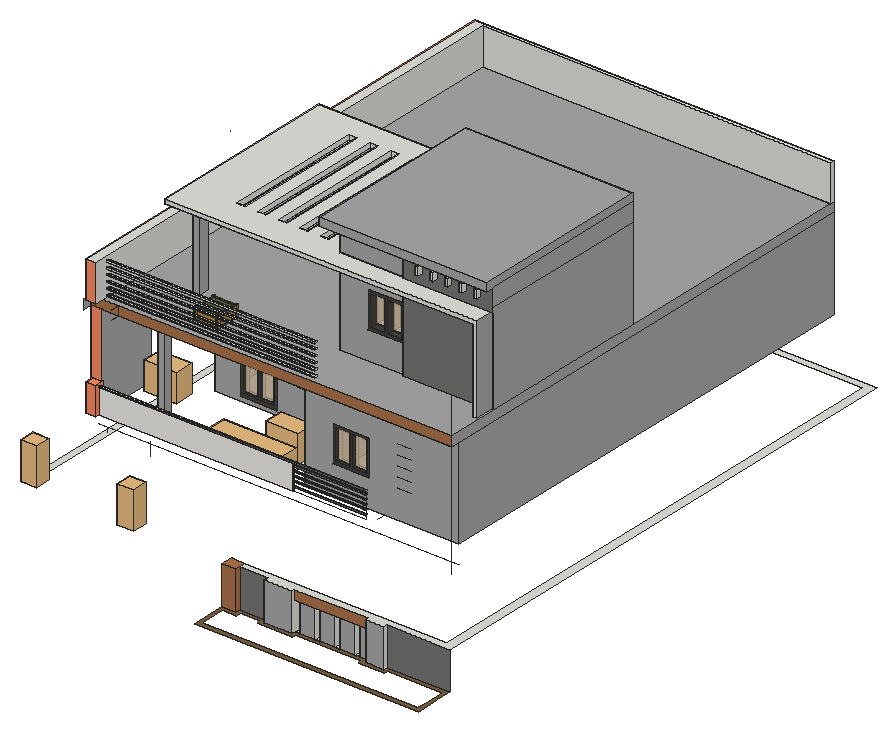
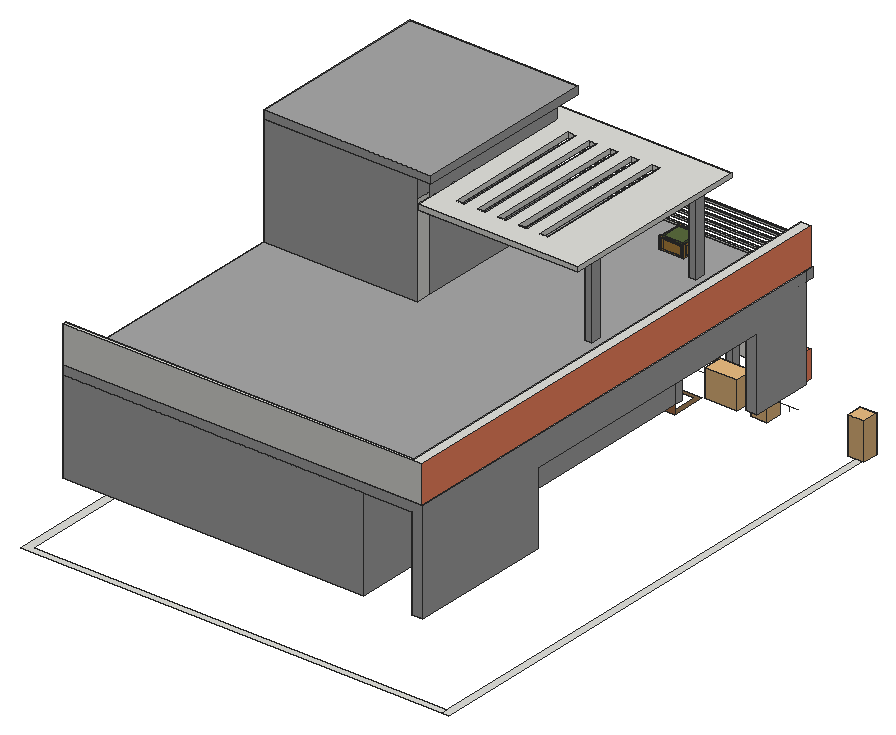
# SketchUp Ruby script. Lengths in inches.
U = 1.inch
M = Sketchup.active_model
def pt(a) = Geom::Point3d.new(a.map { |v| v * U })
def face(e, loops, mat)
  f = e.add_face(loops[0].map { |a| pt(a) })
  loops[1..].each { |l| e.add_face(l.map { |a| pt(a) }).erase! }
  f.material = f.back_material = mat if mat
  f
end
# faces: each face lists its corners as indices into pts; further lists are holes
def faces(e, pts, list, mat = nil) = list.each { |f| face(e, (f[0].is_a?(Array) ? f : [f]).map { |l| l.map { |i| pts[i] } }, mat) }
# xy, xz, yz: faces in a plane at the given z, y or x. An outline is a flat list of corners, or four numbers for a rectangle; further outlines are holes
def ring(l) = l.size == 4 ? [[l[0], l[1]], [l[2], l[1]], [l[2], l[3]], [l[0], l[3]]] : l.each_slice(2).to_a
def flat(e, list, mat, &to3) = list.each { |f| face(e, (f[0].is_a?(Array) ? f : [f]).map { |l| ring(l).map { |u, v| to3.(u, v) } }, mat) }
def xy(e, z, list, mat = nil) = flat(e, list, mat) { |x, y| [x, y, z] }
def xz(e, y, list, mat = nil) = flat(e, list, mat) { |x, z| [x, y, z] }
def yz(e, x, list, mat = nil) = flat(e, list, mat) { |y, z| [x, y, z] }
def lines(e, pts, list) = list.each { |a, b| e.add_line(pt(pts[a]), pt(pts[b])) }
# prism: a flat outline (further loops are holes) pulled along v
def prism(e, loops, v, mat = nil)
  f = face(e, loops, mat); d = Geom::Vector3d.new(v.map { |x| x * U })
  f.pushpull(f.normal.samedirection?(d) ? d.length : -d.length)
end
def box(e, o, s, mat = nil) = prism(e, [[o, [o[0] + s[0], o[1], o[2]], [o[0] + s[0], o[1] + s[1], o[2]], [o[0], o[1] + s[1], o[2]]]], [0, 0, s[2]], mat)
def at(x, y, z, deg = 0) = Geom::Transformation.translation(pt([x, y, z])) * Geom::Transformation.rotation(ORIGIN, Z_AXIS, deg.degrees)
def axes(o, x, y, z) = Geom::Transformation.new([*x, 0, *y, 0, *z, 0, *pt(o).to_a, 1])
def part(name) = M.definitions.add(name)
# library, detail: a bought-in or finely detailed component or shape, given as its bounding box
def library(name, o, s) = part(name).tap { |d| box(d.entities, o, s) }
def detail(e, o, s) = box(e.add_group.entities, o, s)
def put(e, d, t, mat = nil) = e.add_instance(d, t).tap { |i| i.material = mat if mat }
def group(e, t, mat = nil) = e.add_group.tap { |g| g.transformation = t; g.material = mat if mat }.entities
root = M.entities
M.materials.add("!长灌木1").color = [90, 107, 61]
M.materials.add("B03_Apricot_Glow").color = [255, 140, 101]
M.materials.add("Glass_Mirror_01").color = [226, 201, 168]
M.materials["Glass_Mirror_01"].alpha = 0.74
M.materials.add("Image").color = [118, 118, 115]
M.materials.add("M03_Pewter_Shine").color = [168, 168, 168]
M.materials.add("Material20").color = [184, 138, 65]
M.materials.add("Material48").color = [126, 124, 110]
M.materials.add("Metal_06_1K").color = [238, 236, 231]
M.materials.add("Metal_32_1K").color = [117, 124, 125]
M.materials.add("Soil_03_1K").color = [122, 96, 67]
M.materials.add("Wood_Floor_12_1K").color = [45, 37, 32]
M.materials.add("Wood_Planks_01_1K").color = [69, 67, 63]
M.materials.add("Wood_Veneer_15_1K").color = [173, 116, 75]
M.materials.add("Wood_Veneer_15_1K2").color = [173, 116, 75]
c1 = library("Group_2",[-1.28,-0.39,0],[21.22,20.51,48.44])
c2 = library("Planted wooden trough",[0,0,0],[56.02,15.3,25.28])
c3 = library("FF_Model_ID8636_1_ruthrocker1",[-22.29,-12.06,-2.32],[42.44,25.59,36.01])
c4 = part("组\#1")
xy(c4.entities,0,[[0,0,2.36,2.36],[29.92,0,32.28,2.36],[0,29.92,2.36,32.28],[29.92,29.92,32.28,32.28]],"Material48")
xy(c4.entities,1.57,[[2.36,0.39,2.36,2.36,0.39,2.36,0.39,29.92,2.36,29.92,2.36,31.89,29.92,31.89,29.92,29.92,31.89,29.92,31.89,2.36,29.92,2.36,29.92,0.39]],"Material48")
xy(c4.entities,2.76,[[3.54,0.39,28.74,1.57],[0.39,3.54,1.57,28.74],[30.71,3.54,31.89,28.74],[3.54,30.71,28.74,31.89]],"Material20")
xy(c4.entities,20.08,[[3.54,0.39,28.74,1.57],[0.39,3.54,1.57,28.74],[30.71,3.54,31.89,28.74],[3.54,30.71,28.74,31.89]],"Material20")
xy(c4.entities,21.0625,[[2.36,2.36,29.92,29.92]],"!长灌木1")
xy(c4.entities,21.26,[[2.36,0.39,29.92,2.36],[0.39,2.36,2.36,29.92],[29.92,2.36,31.89,29.92],[2.36,29.92,29.92,31.89]],"Material20")
xy(c4.entities,21.38,[[2.36,2.36,29.92,29.92]],"!长灌木1")
xy(c4.entities,22.83,[[0,0,2.36,2.36],[29.92,0,32.28,2.36],[0,29.92,2.36,32.28],[29.92,29.92,32.28,32.28]],"Material20")
xz(c4.entities,0,[[0,0,2.36,22.83],[29.92,0,32.28,22.83]],"Material20")
xz(c4.entities,0.39,[[[2.36,1.57,29.92,21.26],[3.54,2.76,28.74,20.08]]],"Material20")
xz(c4.entities,1.57,[[3.54,2.76,28.74,20.08]],"Material20")
xz(c4.entities,2.36,[[2.36,21.0625,29.92,21.38],[2.36,21.26,29.92,23.43]],"!长灌木1")
xz(c4.entities,2.36,[[0,0,0,22.83,2.36,22.83,2.36,21.26,0.39,21.26,0.39,1.57,2.36,1.57,2.36,0],[29.92,0,29.92,1.57,31.89,1.57,31.89,21.26,29.92,21.26,29.92,22.83,32.28,22.83,32.28,0]],"Material20")
xz(c4.entities,3.54,[[0.39,2.76,1.57,20.08],[30.71,2.76,31.89,20.08]],"Material20")
xz(c4.entities,28.74,[[0.39,2.76,1.57,20.08],[30.71,2.76,31.89,20.08]],"Material20")
xz(c4.entities,29.92,[[2.36,21.0625,29.92,21.38],[2.36,21.26,29.92,23.43]],"!长灌木1")
xz(c4.entities,29.92,[[0,0,2.36,0,2.36,1.57,0.39,1.57,0.39,22.83,0,22.83],[29.92,0,32.28,0,32.28,22.83,31.89,22.83,31.89,1.57,29.92,1.57],[0.39,21.26,2.36,22.83],[29.92,21.26,31.89,22.83]],"Material20")
xz(c4.entities,30.71,[[3.54,2.76,28.74,20.08]],"Material20")
xz(c4.entities,31.89,[[[2.36,1.57,29.92,21.26],[3.54,2.76,28.74,20.08]]],"Material20")
xz(c4.entities,32.28,[[0,0,2.36,22.83],[29.92,0,32.28,22.83]],"Material20")
yz(c4.entities,0,[[0,0,2.36,22.83],[29.92,0,32.28,22.83]],"Material20")
yz(c4.entities,0.39,[[[2.36,1.57,29.92,21.26],[3.54,2.76,28.74,20.08]]],"Material20")
yz(c4.entities,1.57,[[3.54,2.76,28.74,20.08]],"Material20")
yz(c4.entities,2.36,[[0,0,2.36,0,2.36,1.57,0.39,1.57,0.39,22.83,0,22.83]])
yz(c4.entities,2.36,[[2.36,21.0625,29.92,21.38],[2.36,21.26,29.92,23.43]],"!长灌木1")
yz(c4.entities,2.36,[[29.92,0,32.28,0,32.28,22.83,29.92,22.83,29.92,21.26,31.89,21.26,31.89,1.57,29.92,1.57],[0.39,21.26,2.36,22.83]],"Material20")
yz(c4.entities,3.54,[[0.39,2.76,1.57,20.08],[30.71,2.76,31.89,20.08]],"Material20")
yz(c4.entities,28.74,[[0.39,2.76,1.57,20.08],[30.71,2.76,31.89,20.08]],"Material20")
yz(c4.entities,29.92,[[2.36,21.0625,29.92,21.38],[2.36,21.26,29.92,23.43]],"!长灌木1")
yz(c4.entities,29.92,[[0,0,0,22.83,2.36,22.83,2.36,21.26,0.39,21.26,0.39,1.57,2.36,1.57,2.36,0],[29.92,0,29.92,1.57,31.89,1.57,31.89,21.26,29.92,21.26,29.92,22.83,32.28,22.83,32.28,0]],"Material20")
yz(c4.entities,30.71,[[3.54,2.76,28.74,20.08]],"Material20")
yz(c4.entities,31.89,[[[2.36,1.57,29.92,21.26],[3.54,2.76,28.74,20.08]]],"Material20")
yz(c4.entities,32.28,[[0,0,2.36,22.83],[29.92,0,32.28,22.83]],"Material20")
c5 = part("组\#2")
put(c5.entities,c4,at(24.1,23.99,0))
c6 = part("Tree in planter")
put(c6.entities,c5,at(-24.1,-23.99,-1.57))
box(root,[467.44,209.91,404.09],[3.97,6,10.18])
box(root,[486.43,209.91,404.09],[3.97,6,10.18])
box(root,[505.43,209.91,404.09],[3.96,6,10.18])
box(root,[524.42,209.91,404.09],[3.97,6,10.18])
box(root,[543.42,209.91,404.09],[3.96,6,10.18])
xy(root,9.35,[[397.48,100.87,404.48,109.87],[423.47,100.87,430.48,109.87],[449.46,100.87,456.47,109.87],[475.45,100.87,482.46,109.87]])
xy(root,10,[[[307.48,49.75,600.39,49.75,600.39,76.87,600,76.87,600,100.87,517.75,100.87,517.75,95.87,493.75,95.87,493.75,100.87,397.48,100.87,397.48,95.87,361.48,95.87,361.48,100.87,325.48,100.87,325.48,94.87,307.48,94.87],[312.48,54.75,312.48,89.87,330.48,89.87,330.48,95.87,356.48,95.87,356.48,90.87,402.48,90.87,402.48,95.87,488.75,95.87,488.75,90.87,522.75,90.87,522.75,95.87,595,95.87,595,71.87,595.39,71.87,595.39,54.75]]],"Soil_03_1K")
xy(root,48,[[397.48,98.87,397.48,109.87,404.48,109.87,404.48,100.87,423.47,100.87,423.47,109.87,430.48,109.87,430.48,100.87,449.46,100.87,449.46,109.87,456.47,109.87,456.47,100.87,475.45,100.87,475.45,109.87,482.46,109.87,482.46,100.87,493.75,100.87,493.75,98.87]])
xy(root,60,[[361.48,95.87,397.48,95.87,397.48,98.87,493.75,98.87,493.75,95.87,517.75,95.87,517.75,100.87,600,100.87,600,796.87,49.48,796.87,49.48,788.61,588.83,788.61,588.83,109.87,325.48,109.87,325.48,100.87,361.48,100.87],[40.48,100.87,52.41,100.87,52.41,109.87,49.48,109.87,49.48,796.87,40.48,796.87]])
xy(root,60,[[169.48,94.87,187.48,109.87]],"Image")
xy(root,60,[[307.48,94.87,325.48,109.87]],"Wood_Veneer_15_1K2")
xy(root,144,[[95.54,136.48,108.36,149.34],[362.11,141.98,362.74,142.23]],"Metal_06_1K")
xy(root,148.57,[[362.74,142.23,457.3125,142.67],[362.74,142.67,457.3125,143.39]],"Metal_06_1K")
xy(root,149.97,[[362.74,142.23,457.3125,142.67],[362.74,142.67,457.3125,143.39]],"Metal_06_1K")
xy(root,154.62,[[362.74,142.12,457.3125,142.5625],[362.74,142.5625,457.3125,143.27]],"Metal_06_1K")
xy(root,156.02,[[362.74,142.12,457.3125,142.5625],[362.74,142.5625,457.3125,143.27]],"Metal_06_1K")
xy(root,160.67,[[362.74,142.01,457.3125,142.45],[362.74,142.45,457.3125,143.16]],"Metal_06_1K")
xy(root,162.07,[[362.74,142.01,457.3125,142.45],[362.74,142.45,457.3125,143.16]],"Metal_06_1K")
xy(root,166.72,[[362.74,141.9,457.3125,142.34],[362.74,142.34,457.3125,143.05]],"Metal_06_1K")
xy(root,168.125,[[362.74,141.9,457.3125,142.34],[362.74,142.34,457.3125,143.05]],"Metal_06_1K")
xy(root,172.78,[[362.74,141.79,457.3125,142.23],[362.74,142.23,457.3125,142.94]],"Metal_06_1K")
xy(root,174.18,[[362.74,141.79,457.3125,142.23],[362.74,142.23,457.3125,142.94]],"Metal_06_1K")
xy(root,176.97,[[108.36,141.22,457.3125,142.23],[108.36,142.23,457.3125,143.24]],"Metal_06_1K")
xy(root,177.05,[[362.11,141.98,362.74,142.23]],"Metal_06_1K")
xy(root,178.53,[[108.36,141.22,457.3125,143.24]],"Metal_06_1K")
xy(root,180,[[95.54,136.48,108.36,149.34]],"B03_Apricot_Glow")
xy(root,276,[[95.54,136.48,95.54,772.78,564,772.78,564,768.28,108.36,768.28,108.36,136.48],[555,193.91,561,217.91]])
xy(root,277.79,[[108.36,152.97,381.48,156.4]])
xy(root,279.65,[[108.36,152.97,381.48,156.4]])
xy(root,285.92,[[108.36,152.97,381.48,156.4]])
xy(root,287.78,[[108.36,152.97,381.48,156.4]])
xy(root,294.05,[[108.36,152.97,381.48,156.4]])
xy(root,295.9,[[108.36,152.97,381.48,156.4]])
xy(root,302.18,[[108.36,152.97,381.48,156.4]])
xy(root,304.03,[[108.36,152.97,381.48,156.4]])
xy(root,310.31,[[108.36,152.97,381.48,156.4]])
xy(root,312.16,[[108.36,152.97,381.48,156.4]])
xy(root,318.4375,[[108.36,152.97,381.48,156.4]])
xy(root,320.29,[[108.36,152.97,381.48,156.4]])
xy(root,324,[[95.54,136.48,108.36,136.48,108.36,768.28,564,768.28,564,772.78,95.54,772.78]])
xy(root,384.125,[[[153.81,193.91,153.81,444.72,363,444.72,363,217.91,555,217.91,555,193.91],[217.48,231.8,227.53,414.15],[244.73,231.8,254.78,414.15],[271.99,231.8,282.04,414.15],[299.24,231.8,309.29,414.15],[326.49,231.8,336.54,414.15]]])
xy(root,390.125,[[[153.81,193.91,561,193.91,561,217.91,363,217.91,363,444.72,153.81,444.72],[326.49,231.8,336.54,414.15],[299.24,231.8,309.29,414.15],[271.99,231.8,282.04,414.15],[244.73,231.8,254.78,414.15],[217.48,231.8,227.53,414.15]]])
xz(root,94.87,[[307.48,10,325.48,60]],"Wood_Veneer_15_1K2")
xz(root,95.87,[[361.48,10,397.48,60],[493.75,10,517.75,60]],"M03_Pewter_Shine")
xz(root,98.87,[[397.48,48,493.75,60]],"Wood_Veneer_15_1K2")
xz(root,100.87,[[397.48,9.35,404.48,10],[423.47,9.35,430.48,10],[449.46,9.35,456.47,10],[475.45,9.35,482.46,10]])
xz(root,100.87,[[325.48,10,361.48,60],[517.75,10,600,60]],"Image")
xz(root,100.87,[[404.48,10,423.47,48],[430.48,10,449.46,48],[456.47,10,475.45,48],[482.46,10,493.75,48]],"M03_Pewter_Shine")
xz(root,136.48,[[95.54,144,108.36,180],[95.54,276,108.36,324]],"B03_Apricot_Glow")
xz(root,141.22,[[108.36,176.97,457.3125,178.53]],"Metal_32_1K")
xz(root,141.79,[[362.74,172.78,457.3125,174.18]],"Metal_32_1K")
xz(root,141.9,[[362.74,166.72,457.3125,168.125]],"Metal_32_1K")
xz(root,141.98,[[362.11,144,362.74,177.05]],"Metal_32_1K")
xz(root,142.01,[[362.74,160.67,457.3125,162.07]],"Metal_32_1K")
xz(root,142.12,[[362.74,154.62,457.3125,156.02]],"Metal_32_1K")
xz(root,142.23,[[108.36,144,362.11,176.97],[362.11,144,362.73,176.97],[362.73,144,362.74,176.97],[362.11,176.97,362.73,177.05],[362.73,176.97,362.74,177.05]],"Metal_06_1K")
xz(root,142.23,[[362.74,148.57,457.3125,149.97]],"Metal_32_1K")
xz(root,142.94,[[362.74,172.78,457.3125,174.18]],"Metal_06_1K")
xz(root,143.05,[[362.74,166.72,457.3125,168.125]],"Metal_06_1K")
xz(root,143.16,[[362.74,160.67,457.3125,162.07]],"Metal_06_1K")
xz(root,143.24,[[108.36,176.97,457.3125,178.53]],"Metal_06_1K")
xz(root,143.27,[[362.74,154.62,457.3125,156.02]],"Metal_06_1K")
xz(root,143.39,[[362.74,148.57,457.3125,149.97]],"Metal_06_1K")
xz(root,149.34,[[95.54,144,108.36,180]],"Metal_06_1K")
xz(root,152.97,[[108.36,277.79,381.48,279.65],[108.36,285.92,381.48,287.78],[108.36,294.05,381.48,295.9],[108.36,302.18,381.48,304.03],[108.36,310.31,381.48,312.16],
  [108.36,318.4375,381.48,320.29]])
xz(root,156.4,[[108.36,277.79,381.48,279.65],[108.36,285.92,381.48,287.78],[108.36,294.05,381.48,295.9],[108.36,302.18,381.48,304.03],[108.36,310.31,381.48,312.16],
  [108.36,318.4375,381.48,320.29]])
xz(root,193.91,[[555,276,561,276,561,390.125,153.81,390.125,153.81,384.125,555,384.125]])
xz(root,217.91,[[555,276,555,384.125,363,384.125,363,390.125,561,390.125,561,276]])
xz(root,231.8,[[217.48,384.125,227.53,390.125],[244.73,384.125,254.78,390.125],[271.99,384.125,282.04,390.125],[299.24,384.125,309.29,390.125],[326.49,384.125,336.54,390.125]])
xz(root,414.15,[[217.48,384.125,227.53,390.125],[244.73,384.125,254.78,390.125],[271.99,384.125,282.04,390.125],[299.24,384.125,309.29,390.125],[326.49,384.125,336.54,390.125]])
xz(root,444.72,[[153.81,384.125,363,390.125]])
xz(root,768.28,[[108.36,276,564,324]])
xz(root,772.78,[[95.54,276,564,324]])
yz(root,95.54,[[136.48,144,149.34,180],[136.48,276,772.78,324]],"B03_Apricot_Glow")
yz(root,108.36,[[[136.48,276,768.28,324],[152.97,318.4375,156.4,320.29],[152.97,310.31,156.4,312.16],[152.97,302.18,156.4,304.03],[152.97,294.05,156.4,295.9],[152.97,285.92,156.4,287.78],[152.97,277.79,156.4,279.65]]])
yz(root,108.36,[[136.48,144,142.23,144,142.23,176.97,141.22,176.97,141.22,178.53,143.24,178.53,143.24,176.97,142.23,176.97,142.23,144,149.34,144,149.34,180,136.48,180]],"B03_Apricot_Glow")
yz(root,153.81,[[193.91,384.125,444.72,390.125]])
yz(root,217.48,[[231.8,384.125,414.15,390.125]])
yz(root,227.53,[[231.8,384.125,414.15,390.125]])
yz(root,244.73,[[231.8,384.125,414.15,390.125]])
yz(root,254.78,[[231.8,384.125,414.15,390.125]])
yz(root,271.99,[[231.8,384.125,414.15,390.125]])
yz(root,282.04,[[231.8,384.125,414.15,390.125]])
yz(root,299.24,[[231.8,384.125,414.15,390.125]])
yz(root,309.29,[[231.8,384.125,414.15,390.125]])
yz(root,325.48,[[94.87,10,100.87,60]],"Wood_Veneer_15_1K2")
yz(root,326.49,[[231.8,384.125,414.15,390.125]])
yz(root,336.54,[[231.8,384.125,414.15,390.125]])
yz(root,361.48,[[95.87,10,100.87,60]])
yz(root,362.11,[[141.98,144,142.23,177.05]],"Metal_06_1K")
yz(root,362.74,[[141.98,144,142.23,144,142.23,154.62,142.12,154.62,142.12,156.02,142.23,156.02,142.23,160.67,142.01,160.67,142.01,162.07,142.23,162.07,142.23,166.72,141.98,166.72],[142.23,148.57,143.39,149.97],[142.12,154.62,142.23,156.02],[142.23,154.62,143.27,156.02],[142.01,160.67,142.23,162.07],
  [142.23,160.67,143.16,162.07],[141.9,166.72,141.98,168.125],[141.98,166.72,142.23,168.125],[142.23,166.72,143.05,168.125],[141.98,168.125,142.23,172.78],
  [141.79,172.78,141.98,174.18],[141.98,172.78,142.23,174.18],[142.23,172.78,142.94,174.18],[141.98,174.18,142.23,177.05]],"Metal_06_1K")
yz(root,363,[[424.71,276,444.72,384.125],[217.91,384.125,424.71,390.125],[424.71,384.125,444.72,390.125],[424.71,390.125,444.72,396]])
yz(root,381.48,[[152.97,277.79,156.4,279.65],[152.97,285.92,156.4,287.78],[152.97,294.05,156.4,295.9],[152.97,302.18,156.4,304.03],[152.97,310.31,156.4,312.16],
  [152.97,318.4375,156.4,320.29]])
yz(root,397.48,[[100.87,9.35,109.87,9.35,109.87,48,98.87,48,98.87,60,95.87,60,95.87,10,100.87,10]])
yz(root,404.48,[[100.87,9.35,109.87,48]])
yz(root,423.47,[[100.87,9.35,109.87,48]])
yz(root,430.48,[[100.87,9.35,109.87,48]])
yz(root,449.46,[[100.87,9.35,109.87,48]])
yz(root,456.47,[[100.87,9.35,109.87,48]])
yz(root,457.3125,[[141.79,172.78,142.94,174.18],[141.22,176.97,143.24,178.53]],"Metal_06_1K")
yz(root,475.45,[[100.87,9.35,109.87,48]])
yz(root,482.46,[[100.87,9.35,109.87,48]])
yz(root,493.75,[[95.87,10,95.87,60,98.87,60,98.87,48,100.87,48,100.87,10]])
yz(root,517.75,[[95.87,10,100.87,60]])
yz(root,555,[[193.91,276,217.91,384.125]])
yz(root,561,[[193.91,276,217.91,390.125]],"M03_Pewter_Shine")
yz(root,564,[[768.28,276,772.78,324]])
p = [[564,160.87,120],[104.42,160.87,120],[466.47,148.87,144],[466.47,160.87,144],[558,148.87,324],[564,148.87,324],
  [564,148.87,114],[457.3125,142.23,176.97],[457.3125,142.23,174.18],[457.3125,142.23,144],[362.74,142.23,144],[457.3125,142.23,172.78],
  [457.3125,142.23,168.125],[457.3125,142.23,166.72],[457.3125,142.23,162.07],[457.3125,142.23,160.67],[457.3125,142.23,156.02],[457.3125,142.23,154.62],
  [457.3125,142.23,149.97],[457.3125,142.23,148.57],[107.42,160.87,264],[107.42,772.87,264],[170.58,148.87,114],[170.58,148.87,132],
  [93,160.87,120],[104.42,160.87,114],[492.53,148.87,242.0625],[510.62,148.87,242.0625],[492.53,148.87,229.11],[510.62,148.87,229.11],
  [492.53,148.87,216.16],[510.62,148.87,216.16],[492.53,148.87,203.21],[510.62,148.87,203.21],[492.53,148.87,190.26],[510.62,148.87,190.26]]
lines(root,p,[[0,1],[2,3],[4,5],[5,6],[7,8],[9,10],[11,12],[13,14],[12,13],[15,16],[14,15],[17,18],
  [16,17],[19,9],[20,21],[22,23],[1,24],[25,1],[26,27],[28,29],[30,31],[32,33],[34,35]])
put(root,c1,at(171.67,94.87,57.68))
put(root,c1,at(40.48,100.87,60))
put(root,c2,axes([241.96,154.9,144],[1.6992,0,0],[0,1.57,0],[0,0,1]))
put(root,c3,at(312.11,199.63,146.32))
put(root,c3,at(135.61,221.67,146.32))
g1 = group(root,at(129,160.87,144),"M03_Pewter_Shine")
xy(g1,0,[[243,9,426,93],[51,102,426,603]])
xy(g1,10,[[97.375,93,96.8,97.5,96.22,102,100.22,102,100.8,97.5,101.375,93],[79,97.5,96.8,97.5,96.22,102,79,102],[100.8,97.5,119,97.5,119,102,100.22,102]])
xy(g1,10,[[79,93,97.375,93,96.8,97.5,79,97.5],[101.375,93,119,93,119,97.5,100.8,97.5]],"Wood_Planks_01_1K")
xy(g1,40,[[274,4.5,292,9],[296,4.5,314,9]])
xy(g1,40,[[274,0,292,4.5],[296,0,314,4.5]],"Wood_Planks_01_1K")
xy(g1,46,[[151,97.5,169,102],[173,97.5,191,102]])
xy(g1,46,[[151,93,169,97.5],[173,93,191,97.5]],"Wood_Planks_01_1K")
xy(g1,80,[[274,4.5,292,9],[296,4.5,314,9]])
xy(g1,80,[[274,0,292,4.5],[296,0,314,4.5]],"Wood_Planks_01_1K")
xy(g1,86,[[79,97.5,79,102,96.22,102,96.8,97.5],[100.8,97.5,100.22,102,119,102,119,97.5],[151,97.5,169,102],[173,97.5,191,102]])
xy(g1,86,[[79,93,79,97.5,96.8,97.5,97.375,93],[101.375,93,100.8,97.5,119,97.5,119,93],[151,93,169,97.5],[173,93,191,97.5]],"Wood_Planks_01_1K")
xy(g1,120,[[41.58,0,50.58,10],[234,0,435,0,435,612,42,612,42,603,426,603,426,9,243,9,243,93,234,93],[41.58,93,42,102],[42,93,51,603],[51,93,426,102]])
xz(g1,0,[[41.58,0,50.58,120],[[234,0,435,120],[270,36,318,84]]])
xz(g1,0,[[[270,36,318,84],[274,40,292,80],[296,40,314,80]]],"Wood_Planks_01_1K")
xz(g1,4.5,[[274,40,292,80],[296,40,314,80]],"Glass_Mirror_01")
xz(g1,9,[[[243,0,426,120],[274,40,292,80],[296,40,314,80]]])
xz(g1,10,[[41.58,0,50.58,120]])
xz(g1,93,[[41.58,0,42,120,41.58,120],[[41.58,0,234,0,234,120,42,120],[75,6,123,90],[147,42,195,90]],[234,0,243,120],[243,0,426,120]])
xz(g1,93,[[[75,6,123,90],[79,10,97.375,86],[101.375,10,119,86]],[[147,42,195,90],[151,46,169,86],[173,46,191,86]]],"Wood_Planks_01_1K")
xz(g1,97.5,[[79,10,96.8,86],[100.8,10,119,86],[151,46,169,86],[173,46,191,86]],"Glass_Mirror_01")
xz(g1,102,[[41.58,0,42,120],[[51,0,426,120],[100.22,10,119,86],[79,10,96.22,86],[151,46,169,86],[173,46,191,86]]])
xz(g1,603,[[51,0,396,120],[396,0,426,120]])
xz(g1,612,[[42,0,435,120]])
yz(g1,41.58,[[0,0,10,120],[93,0,102,120]])
yz(g1,42,[[102,0,612,120]])
yz(g1,50.58,[[0,0,10,120]])
yz(g1,51,[[102,0,603,120]])
yz(g1,79,[[97.5,10,102,86]])
yz(g1,79,[[93,10,97.5,86]],"Wood_Planks_01_1K")
yz(g1,119,[[97.5,10,102,86]])
yz(g1,119,[[93,10,97.5,86]],"Wood_Planks_01_1K")
yz(g1,151,[[97.5,46,102,86]])
yz(g1,151,[[93,46,97.5,86]],"Wood_Planks_01_1K")
yz(g1,169,[[97.5,46,102,86]])
yz(g1,169,[[93,46,97.5,86]],"Wood_Planks_01_1K")
yz(g1,173,[[97.5,46,102,86]])
yz(g1,173,[[93,46,97.5,86]],"Wood_Planks_01_1K")
yz(g1,191,[[97.5,46,102,86]])
yz(g1,191,[[93,46,97.5,86]],"Wood_Planks_01_1K")
yz(g1,234,[[0,0,93,120]])
yz(g1,243,[[9,0,93,120]])
yz(g1,274,[[4.5,40,9,80]])
yz(g1,274,[[0,40,4.5,80]],"Wood_Planks_01_1K")
yz(g1,292,[[4.5,40,9,80]])
yz(g1,292,[[0,40,4.5,80]],"Wood_Planks_01_1K")
yz(g1,296,[[4.5,40,9,80]])
yz(g1,296,[[0,40,4.5,80]],"Wood_Planks_01_1K")
yz(g1,314,[[4.5,40,9,80]])
yz(g1,314,[[0,40,4.5,80]],"Wood_Planks_01_1K")
yz(g1,426,[[9,0,93,120],[93,0,102,120],[102,0,603,120]])
yz(g1,435,[[0,0,612,120]])
p = [[97.375,93,86],[96.8,97.5,86],[96.8,97.5,10],[97.375,93,10],[101.375,93,10],[100.8,97.5,10],
  [100.8,97.5,86],[101.375,93,86],[96.22,102,10],[96.22,102,86],[100.22,102,86],[100.22,102,10],
  [42,603,0],[51,603,0]]
faces(g1,p,[[0,1,2,3],[4,5,6,7]],"Wood_Planks_01_1K")
faces(g1,p,[[8,2,1,9],[10,6,5,11]])
lines(g1,p,[[12,13]])
g2 = group(root,at(129,160.87,264),"M03_Pewter_Shine")
xy(g2,-120,[[-36,-12.24,-21.58,67.85],[-36,425.43,-21.58,612]])
xy(g2,0,[[-36,-12.24,-21.58,-12.24,-36,-12.19]])
xy(g2,0,[[-21.58,-12.24,-21.58,0,0,-12.24],[0,-12.24,-21.58,0,-21.58,612,435,612,435,-12.24]],"Wood_Floor_12_1K")
xy(g2,12,[[-36,-12.24,435,612]])
xz(g2,-12.24,[[-36,-120,-21.58,0]],"B03_Apricot_Glow")
xz(g2,-12.24,[[-36,0,0,12],[0,0,435,12]],"Wood_Veneer_15_1K")
xz(g2,67.85,[[-36,-120,-21.58,-25.97]])
xz(g2,425.43,[[-36,-120,-21.58,-111.33],[-36,-111.33,-21.58,-25.22]])
xz(g2,612,[[-36,-120,-36,12,435,12,435,0,-21.58,0,-21.58,-120]])
yz(g2,-36,[[-12.24,-120,-12.24,12,612,12,612,-120,425.43,-120,425.43,-25.22,67.85,-25.97,67.85,-120],[-24.39,0,-12.24,12]])
yz(g2,-21.58,[[-12.24,-120,67.85,-120,67.85,-25.97,425.43,-25.22,425.43,-120,612,-120,612,0,-12.24,0]])
yz(g2,435,[[-12.24,0,612,12]])
p = [[-36,67.85,-25.97],[-36,425.43,-25.22],[-21.58,425.43,-25.22],[-21.58,67.85,-25.97],[234,-12.24,0],[234,93,0],
  [-36,-12.19,0],[-36,-11.25,0],[-36,0,0],[-21.58,0,0],[0,-12.24,12],[0,-24.39,12],
  [0,-24.39,0],[0,-12.24,0]]
faces(g2,p,[[0,1,2,3]])
lines(g2,p,[[4,5],[6,7],[8,9],[10,11],[12,13]])
put(root,c6,axes([207.34,172.76,276],[1,0,0],[0,1,0],[0,0,0.73495]))
g3 = group(root,at(95.81,93.58,288),"M03_Pewter_Shine")
xy(g3,-12,[[351.19,122.34,459.19,122.34,459.19,124.34,468.19,124.34,468.19,351.14,459.19,351.14,459.19,144.35,276.19,144.35,276.19,331.13,267.19,331.13,267.19,124.34,351.19,124.34],[276.19,144.35,459.19,331.13]])
xy(g3,28,[[307.19,134.34,325.19,144.35],[329.19,134.34,347.19,144.35]])
xy(g3,28,[[307.19,124.34,325.19,134.34],[329.19,124.34,347.19,134.34]],"Wood_Planks_01_1K")
xy(g3,68,[[307.19,134.34,325.19,144.35],[329.19,134.34,347.19,144.35]])
xy(g3,68,[[307.19,124.34,325.19,134.34],[329.19,124.34,347.19,134.34]],"Wood_Planks_01_1K")
xy(g3,96.125,[[351.19,122.34,459.19,124.34],[74.77,124.34,83.77,137.97]])
xy(g3,102.125,[[351.19,122.34,468.19,124.34]])
xy(g3,132,[[[351.19,122.34,468.19,122.34,468.19,351.14,267.19,351.14,267.19,124.34,351.19,124.34],[276.19,144.35,459.19,331.13]]])
xz(g3,122.34,[[351.19,-12,459.19,96.125],[351.19,102.125,468.19,132]],"Image")
xz(g3,124.34,[[74.77,-12,83.77,96.125],[267.19,-12,351.19,-12,351.19,24,303.19,24,303.19,72,351.19,72,351.19,132,267.19,132],[459.19,-12,468.19,-12,468.19,102.125,351.19,102.125,351.19,96.125,459.19,96.125]])
xz(g3,124.34,[[[303.19,24,351.19,72],[307.19,28,325.19,68],[329.19,28,347.19,68]]],"Wood_Planks_01_1K")
xz(g3,134.34,[[307.19,28,325.19,68],[329.19,28,347.19,68]],"Glass_Mirror_01")
xz(g3,137.97,[[74.77,-12,83.77,96.125]])
xz(g3,144.35,[[[276.19,-12,459.19,132],[307.19,28,325.19,68],[329.19,28,347.19,68]]])
xz(g3,293.29,[[74.77,-12,83.77,96.125]])
xz(g3,306.92,[[74.77,-12,83.77,96.125]])
xz(g3,331.13,[[267.19,-12,276.19,108],[276.19,-12,459.19,132]])
xz(g3,351.14,[[267.19,-12,468.19,132]])
yz(g3,74.77,[[124.34,-12,137.97,96.125],[293.29,-12,306.92,96.125]])
yz(g3,83.77,[[124.34,-12,137.97,96.125],[293.29,-12,306.92,96.125]])
yz(g3,267.19,[[124.34,-12,331.13,132],[331.13,108,351.14,132]])
yz(g3,276.19,[[144.35,-12,331.13,132]])
yz(g3,307.19,[[134.34,28,144.35,68]])
yz(g3,307.19,[[124.34,28,134.34,68]],"Wood_Planks_01_1K")
yz(g3,325.19,[[134.34,28,144.35,68]])
yz(g3,325.19,[[124.34,28,134.34,68]],"Wood_Planks_01_1K")
yz(g3,329.19,[[134.34,28,144.35,68]])
yz(g3,329.19,[[124.34,28,134.34,68]],"Wood_Planks_01_1K")
yz(g3,347.19,[[134.34,28,144.35,68]])
yz(g3,347.19,[[124.34,28,134.34,68]],"Wood_Planks_01_1K")
yz(g3,351.19,[[122.34,-12,124.34,24],[122.34,24,124.34,72],[122.34,72,124.34,96.125],[122.34,102.125,124.34,132]])
yz(g3,459.19,[[122.34,-12,124.34,96.125],[144.35,-12,331.13,132]])
yz(g3,468.19,[[124.34,-12,351.14,-12,351.14,108,122.34,108,122.34,102.125,124.34,102.125],[122.34,108,351.14,132]])
p = [[41.58,226.81,120],[42,226.81,120]]
lines(g3,p,[[0,1]])
g4 = group(root,at(363,217.91,420),"M03_Pewter_Shine")
box(g4,[-18,-12,0],[219,238.81,10])
